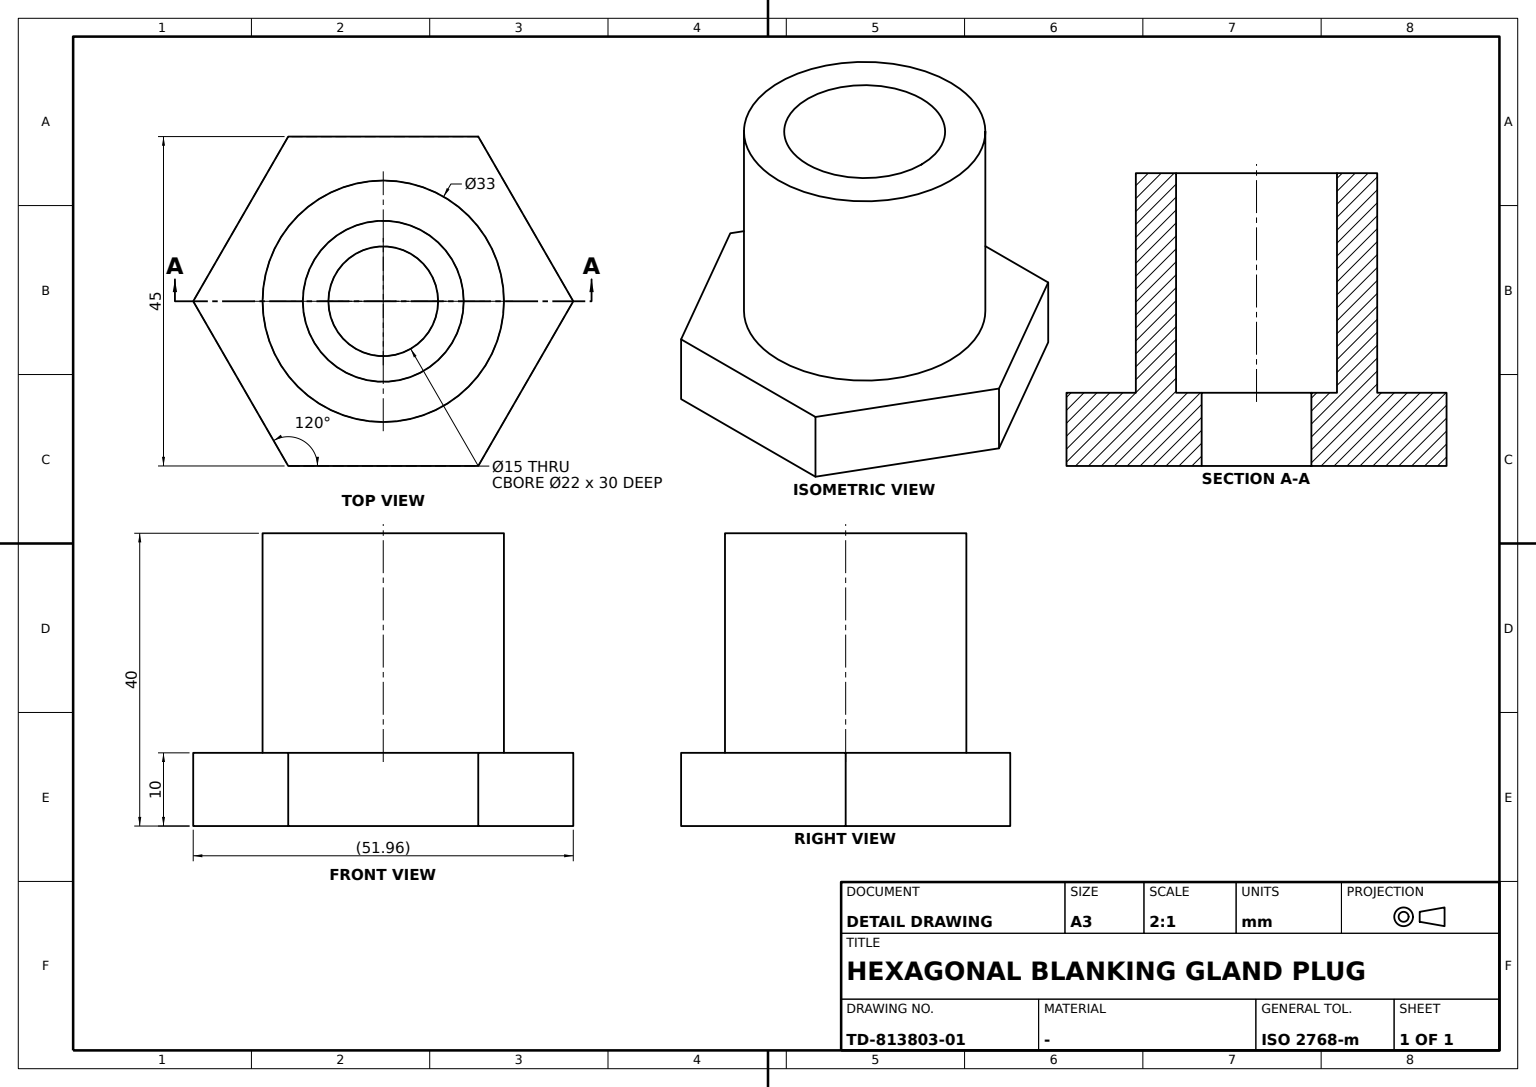
ISO-10303-21;
HEADER;
FILE_DESCRIPTION((''),'2;1');
FILE_NAME('','',(''),(''),'','','');
FILE_SCHEMA(('AUTOMOTIVE_DESIGN'));
ENDSEC;
DATA;
#1=APPLICATION_CONTEXT('');
#2=PRODUCT_CONTEXT('',#1,'mechanical');
#3=PRODUCT('','','',(#2));
#4=PRODUCT_DEFINITION_FORMATION('','',#3);
#5=PRODUCT_DEFINITION_CONTEXT('',#1,'design');
#6=PRODUCT_DEFINITION('','',#4,#5);
#7=PRODUCT_DEFINITION_SHAPE('','',#6);
#8=(LENGTH_UNIT()NAMED_UNIT(*)SI_UNIT(.MILLI.,.METRE.));
#9=(NAMED_UNIT(*)PLANE_ANGLE_UNIT()SI_UNIT($,.RADIAN.));
#10=(NAMED_UNIT(*)SI_UNIT($,.STERADIAN.)SOLID_ANGLE_UNIT());
#11=UNCERTAINTY_MEASURE_WITH_UNIT(LENGTH_MEASURE(0.005),#8,'distance_accuracy_value','');
#12=(GEOMETRIC_REPRESENTATION_CONTEXT(3)GLOBAL_UNCERTAINTY_ASSIGNED_CONTEXT((#11))GLOBAL_UNIT_ASSIGNED_CONTEXT((#8,#9,#10))REPRESENTATION_CONTEXT('',''));
#13=CARTESIAN_POINT('',(12.990381,-22.5,0.));
#14=VERTEX_POINT('',#13);
#15=CARTESIAN_POINT('',(12.990381,-22.5,10.));
#16=VERTEX_POINT('',#15);
#17=DIRECTION('',(0.,0.,1.));
#18=VECTOR('',#17,1000.);
#19=LINE('',#13,#18);
#20=EDGE_CURVE('',#14,#16,#19,.T.);
#21=ORIENTED_EDGE('',*,*,#20,.T.);
#22=CARTESIAN_POINT('',(-12.990381,-22.5,10.));
#23=VERTEX_POINT('',#22);
#24=CARTESIAN_POINT('',(0.,-22.5,10.));
#25=DIRECTION('',(1.,0.,0.));
#26=VECTOR('',#25,1000.);
#27=LINE('',#24,#26);
#28=EDGE_CURVE('',#23,#16,#27,.T.);
#29=ORIENTED_EDGE('',*,*,#28,.F.);
#30=CARTESIAN_POINT('',(-12.990381,-22.5,0.));
#31=VERTEX_POINT('',#30);
#32=LINE('',#30,#18);
#33=EDGE_CURVE('',#31,#23,#32,.T.);
#34=ORIENTED_EDGE('',*,*,#33,.F.);
#35=CARTESIAN_POINT('',(0.,-22.5,0.));
#36=LINE('',#35,#26);
#37=EDGE_CURVE('',#31,#14,#36,.T.);
#38=ORIENTED_EDGE('',*,*,#37,.T.);
#39=EDGE_LOOP('',(#21,#29,#34,#38));
#40=FACE_BOUND('',#39,.T.);
#41=DIRECTION('',(0.,-1.,0.));
#42=AXIS2_PLACEMENT_3D('',#30,#41,#25);
#43=PLANE('',#42);
#44=ADVANCED_FACE('',(#40),#43,.T.);
#45=CARTESIAN_POINT('',(-25.980762,0.,10.));
#46=VERTEX_POINT('',#45);
#47=CARTESIAN_POINT('',(-19.485572,-11.25,10.));
#48=DIRECTION('',(0.5,-0.866025404,0.));
#49=VECTOR('',#48,1000.);
#50=LINE('',#47,#49);
#51=EDGE_CURVE('',#46,#23,#50,.T.);
#52=ORIENTED_EDGE('',*,*,#51,.F.);
#53=CARTESIAN_POINT('',(-25.980762,0.,0.));
#54=VERTEX_POINT('',#53);
#55=LINE('',#53,#18);
#56=EDGE_CURVE('',#54,#46,#55,.T.);
#57=ORIENTED_EDGE('',*,*,#56,.F.);
#58=CARTESIAN_POINT('',(-19.485572,-11.25,0.));
#59=LINE('',#58,#49);
#60=EDGE_CURVE('',#54,#31,#59,.T.);
#61=ORIENTED_EDGE('',*,*,#60,.T.);
#62=ORIENTED_EDGE('',*,*,#33,.T.);
#63=EDGE_LOOP('',(#52,#57,#61,#62));
#64=FACE_BOUND('',#63,.T.);
#65=DIRECTION('',(-0.866025404,-0.5,0.));
#66=AXIS2_PLACEMENT_3D('',#53,#65,#48);
#67=PLANE('',#66);
#68=ADVANCED_FACE('',(#64),#67,.T.);
#69=CARTESIAN_POINT('',(12.990381,22.5,10.));
#70=VERTEX_POINT('',#69);
#71=CARTESIAN_POINT('',(-12.990381,22.5,10.));
#72=VERTEX_POINT('',#71);
#73=CARTESIAN_POINT('',(0.,22.5,10.));
#74=DIRECTION('',(-1.,0.,0.));
#75=VECTOR('',#74,1000.);
#76=LINE('',#73,#75);
#77=EDGE_CURVE('',#70,#72,#76,.T.);
#78=ORIENTED_EDGE('',*,*,#77,.T.);
#79=CARTESIAN_POINT('',(-19.485572,11.25,10.));
#80=DIRECTION('',(-0.5,-0.866025404,0.));
#81=VECTOR('',#80,1000.);
#82=LINE('',#79,#81);
#83=EDGE_CURVE('',#72,#46,#82,.T.);
#84=ORIENTED_EDGE('',*,*,#83,.T.);
#85=ORIENTED_EDGE('',*,*,#51,.T.);
#86=ORIENTED_EDGE('',*,*,#28,.T.);
#87=CARTESIAN_POINT('',(25.980762,0.,10.));
#88=VERTEX_POINT('',#87);
#89=CARTESIAN_POINT('',(19.485572,-11.25,10.));
#90=DIRECTION('',(0.5,0.866025404,0.));
#91=VECTOR('',#90,1000.);
#92=LINE('',#89,#91);
#93=EDGE_CURVE('',#16,#88,#92,.T.);
#94=ORIENTED_EDGE('',*,*,#93,.T.);
#95=CARTESIAN_POINT('',(19.485572,11.25,10.));
#96=DIRECTION('',(-0.5,0.866025404,0.));
#97=VECTOR('',#96,1000.);
#98=LINE('',#95,#97);
#99=EDGE_CURVE('',#88,#70,#98,.T.);
#100=ORIENTED_EDGE('',*,*,#99,.T.);
#101=EDGE_LOOP('',(#78,#84,#85,#86,#94,#100));
#102=FACE_BOUND('',#101,.T.);
#103=CARTESIAN_POINT('',(16.5,0.,10.));
#104=VERTEX_POINT('',#103);
#105=CARTESIAN_POINT('',(0.,0.,10.));
#106=AXIS2_PLACEMENT_3D('',#105,#17,#25);
#107=CIRCLE('',#106,16.5);
#108=EDGE_CURVE('',#104,#104,#107,.T.);
#109=ORIENTED_EDGE('',*,*,#108,.F.);
#110=EDGE_LOOP('',(#109));
#111=FACE_BOUND('',#110,.T.);
#112=PLANE('',#106);
#113=ADVANCED_FACE('',(#102,#111),#112,.T.);
#114=CARTESIAN_POINT('',(7.5,0.,10.));
#115=VERTEX_POINT('',#114);
#116=CIRCLE('',#106,7.5);
#117=EDGE_CURVE('',#115,#115,#116,.T.);
#118=ORIENTED_EDGE('',*,*,#117,.F.);
#119=EDGE_LOOP('',(#118));
#120=FACE_BOUND('',#119,.T.);
#121=CARTESIAN_POINT('',(11.,0.,10.));
#122=VERTEX_POINT('',#121);
#123=CIRCLE('',#106,11.);
#124=EDGE_CURVE('',#122,#122,#123,.T.);
#125=ORIENTED_EDGE('',*,*,#124,.T.);
#126=EDGE_LOOP('',(#125));
#127=FACE_BOUND('',#126,.T.);
#128=ADVANCED_FACE('',(#120,#127),#112,.T.);
#129=CARTESIAN_POINT('',(11.,0.,40.));
#130=VERTEX_POINT('',#129);
#131=CARTESIAN_POINT('',(0.,0.,40.));
#132=AXIS2_PLACEMENT_3D('',#131,#17,#25);
#133=CIRCLE('',#132,11.);
#134=EDGE_CURVE('',#130,#130,#133,.T.);
#135=ORIENTED_EDGE('',*,*,#134,.T.);
#136=EDGE_LOOP('',(#135));
#137=FACE_BOUND('',#136,.T.);
#138=ORIENTED_EDGE('',*,*,#124,.F.);
#139=EDGE_LOOP('',(#138));
#140=FACE_BOUND('',#139,.T.);
#141=CARTESIAN_POINT('',(0.,0.,25.));
#142=AXIS2_PLACEMENT_3D('',#141,#17,#25);
#143=CYLINDRICAL_SURFACE('',#142,11.);
#144=ADVANCED_FACE('',(#137,#140),#143,.F.);
#145=ORIENTED_EDGE('',*,*,#134,.F.);
#146=EDGE_LOOP('',(#145));
#147=FACE_BOUND('',#146,.T.);
#148=CARTESIAN_POINT('',(16.5,0.,40.));
#149=VERTEX_POINT('',#148);
#150=CIRCLE('',#132,16.5);
#151=EDGE_CURVE('',#149,#149,#150,.T.);
#152=ORIENTED_EDGE('',*,*,#151,.T.);
#153=EDGE_LOOP('',(#152));
#154=FACE_BOUND('',#153,.T.);
#155=PLANE('',#132);
#156=ADVANCED_FACE('',(#147,#154),#155,.T.);
#157=ORIENTED_EDGE('',*,*,#151,.F.);
#158=EDGE_LOOP('',(#157));
#159=FACE_BOUND('',#158,.T.);
#160=ORIENTED_EDGE('',*,*,#108,.T.);
#161=EDGE_LOOP('',(#160));
#162=FACE_BOUND('',#161,.T.);
#163=CYLINDRICAL_SURFACE('',#142,16.5);
#164=ADVANCED_FACE('',(#159,#162),#163,.T.);
#165=CARTESIAN_POINT('',(-12.990381,22.5,0.));
#166=VERTEX_POINT('',#165);
#167=LINE('',#165,#18);
#168=EDGE_CURVE('',#166,#72,#167,.T.);
#169=ORIENTED_EDGE('',*,*,#168,.F.);
#170=CARTESIAN_POINT('',(-19.485572,11.25,0.));
#171=LINE('',#170,#81);
#172=EDGE_CURVE('',#166,#54,#171,.T.);
#173=ORIENTED_EDGE('',*,*,#172,.T.);
#174=ORIENTED_EDGE('',*,*,#56,.T.);
#175=ORIENTED_EDGE('',*,*,#83,.F.);
#176=EDGE_LOOP('',(#169,#173,#174,#175));
#177=FACE_BOUND('',#176,.T.);
#178=DIRECTION('',(-0.866025404,0.5,0.));
#179=AXIS2_PLACEMENT_3D('',#165,#178,#80);
#180=PLANE('',#179);
#181=ADVANCED_FACE('',(#177),#180,.T.);
#182=CARTESIAN_POINT('',(25.980762,0.,0.));
#183=VERTEX_POINT('',#182);
#184=CARTESIAN_POINT('',(12.990381,22.5,0.));
#185=VERTEX_POINT('',#184);
#186=CARTESIAN_POINT('',(19.485572,11.25,0.));
#187=LINE('',#186,#97);
#188=EDGE_CURVE('',#183,#185,#187,.T.);
#189=ORIENTED_EDGE('',*,*,#188,.T.);
#190=LINE('',#184,#18);
#191=EDGE_CURVE('',#185,#70,#190,.T.);
#192=ORIENTED_EDGE('',*,*,#191,.T.);
#193=ORIENTED_EDGE('',*,*,#99,.F.);
#194=LINE('',#182,#18);
#195=EDGE_CURVE('',#183,#88,#194,.T.);
#196=ORIENTED_EDGE('',*,*,#195,.F.);
#197=EDGE_LOOP('',(#189,#192,#193,#196));
#198=FACE_BOUND('',#197,.T.);
#199=DIRECTION('',(0.866025404,0.5,0.));
#200=AXIS2_PLACEMENT_3D('',#182,#199,#96);
#201=PLANE('',#200);
#202=ADVANCED_FACE('',(#198),#201,.T.);
#203=ORIENTED_EDGE('',*,*,#168,.T.);
#204=ORIENTED_EDGE('',*,*,#77,.F.);
#205=ORIENTED_EDGE('',*,*,#191,.F.);
#206=CARTESIAN_POINT('',(0.,22.5,0.));
#207=LINE('',#206,#75);
#208=EDGE_CURVE('',#185,#166,#207,.T.);
#209=ORIENTED_EDGE('',*,*,#208,.T.);
#210=EDGE_LOOP('',(#203,#204,#205,#209));
#211=FACE_BOUND('',#210,.T.);
#212=DIRECTION('',(0.,1.,0.));
#213=AXIS2_PLACEMENT_3D('',#184,#212,#74);
#214=PLANE('',#213);
#215=ADVANCED_FACE('',(#211),#214,.T.);
#216=ORIENTED_EDGE('',*,*,#195,.T.);
#217=ORIENTED_EDGE('',*,*,#93,.F.);
#218=ORIENTED_EDGE('',*,*,#20,.F.);
#219=CARTESIAN_POINT('',(19.485572,-11.25,0.));
#220=LINE('',#219,#91);
#221=EDGE_CURVE('',#14,#183,#220,.T.);
#222=ORIENTED_EDGE('',*,*,#221,.T.);
#223=EDGE_LOOP('',(#216,#217,#218,#222));
#224=FACE_BOUND('',#223,.T.);
#225=DIRECTION('',(0.866025404,-0.5,0.));
#226=AXIS2_PLACEMENT_3D('',#13,#225,#90);
#227=PLANE('',#226);
#228=ADVANCED_FACE('',(#224),#227,.T.);
#229=ORIENTED_EDGE('',*,*,#188,.F.);
#230=ORIENTED_EDGE('',*,*,#221,.F.);
#231=ORIENTED_EDGE('',*,*,#37,.F.);
#232=ORIENTED_EDGE('',*,*,#60,.F.);
#233=ORIENTED_EDGE('',*,*,#172,.F.);
#234=ORIENTED_EDGE('',*,*,#208,.F.);
#235=EDGE_LOOP('',(#229,#230,#231,#232,#233,#234));
#236=FACE_BOUND('',#235,.T.);
#237=CARTESIAN_POINT('',(7.5,0.,0.));
#238=VERTEX_POINT('',#237);
#239=CARTESIAN_POINT('',(0.,0.,0.));
#240=AXIS2_PLACEMENT_3D('',#239,#17,#25);
#241=CIRCLE('',#240,7.5);
#242=EDGE_CURVE('',#238,#238,#241,.T.);
#243=ORIENTED_EDGE('',*,*,#242,.T.);
#244=EDGE_LOOP('',(#243));
#245=FACE_BOUND('',#244,.T.);
#246=PLANE('',#240);
#247=ADVANCED_FACE('',(#236,#245),#246,.F.);
#248=ORIENTED_EDGE('',*,*,#117,.T.);
#249=EDGE_LOOP('',(#248));
#250=FACE_BOUND('',#249,.T.);
#251=ORIENTED_EDGE('',*,*,#242,.F.);
#252=EDGE_LOOP('',(#251));
#253=FACE_BOUND('',#252,.T.);
#254=CARTESIAN_POINT('',(0.,0.,-5.));
#255=AXIS2_PLACEMENT_3D('',#254,#17,#25);
#256=CYLINDRICAL_SURFACE('',#255,7.5);
#257=ADVANCED_FACE('',(#250,#253),#256,.F.);
#258=CLOSED_SHELL('',(#44,#68,#113,#128,#144,#156,#164,#181,#202,#215,#228,#247,#257));
#259=MANIFOLD_SOLID_BREP('',#258);
#260=ADVANCED_BREP_SHAPE_REPRESENTATION('',(#259),#12);
#261=SHAPE_DEFINITION_REPRESENTATION(#7,#260);
ENDSEC;
END-ISO-10303-21;
